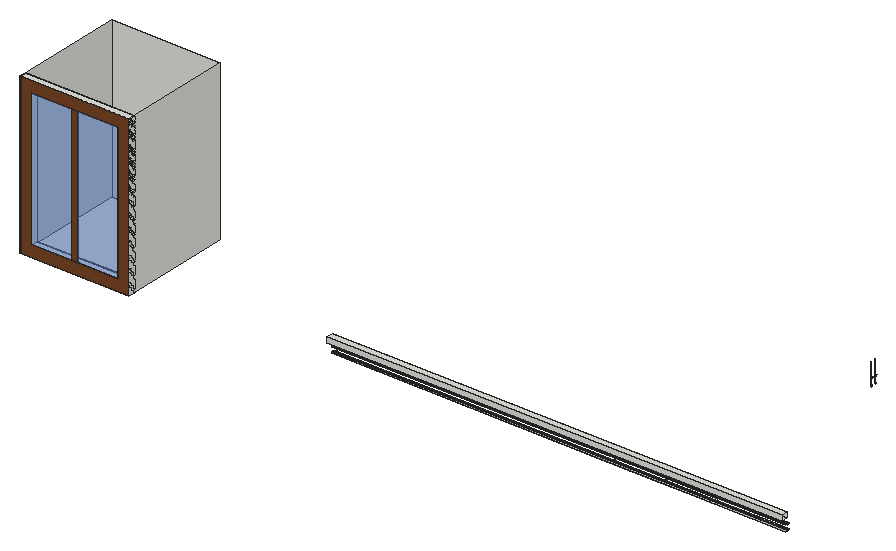
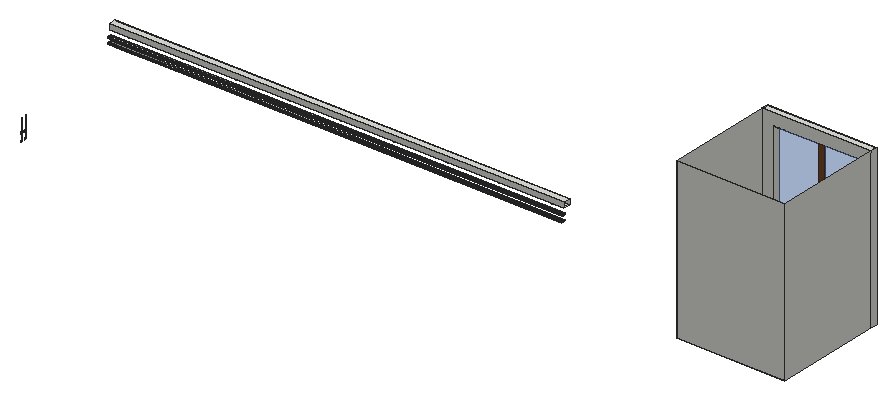
# SketchUp Ruby script. Lengths in inches.
U = 1.inch
M = Sketchup.active_model
def pt(a) = Geom::Point3d.new(a.map { |v| v * U })
def face(e, loops, mat)
  f = e.add_face(loops[0].map { |a| pt(a) })
  loops[1..].each { |l| e.add_face(l.map { |a| pt(a) }).erase! }
  f.material = f.back_material = mat if mat
  f
end
# faces: each face lists its corners as indices into pts; further lists are holes
def faces(e, pts, list, mat = nil) = list.each { |f| face(e, (f[0].is_a?(Array) ? f : [f]).map { |l| l.map { |i| pts[i] } }, mat) }
# xy, xz, yz: faces in a plane at the given z, y or x. An outline is a flat list of corners, or four numbers for a rectangle; further outlines are holes
def ring(l) = l.size == 4 ? [[l[0], l[1]], [l[2], l[1]], [l[2], l[3]], [l[0], l[3]]] : l.each_slice(2).to_a
def flat(e, list, mat, &to3) = list.each { |f| face(e, (f[0].is_a?(Array) ? f : [f]).map { |l| ring(l).map { |u, v| to3.(u, v) } }, mat) }
def xy(e, z, list, mat = nil) = flat(e, list, mat) { |x, y| [x, y, z] }
def xz(e, y, list, mat = nil) = flat(e, list, mat) { |x, z| [x, y, z] }
def yz(e, x, list, mat = nil) = flat(e, list, mat) { |y, z| [x, y, z] }
def lines(e, pts, list) = list.each { |a, b| e.add_line(pt(pts[a]), pt(pts[b])) }
# prism: a flat outline (further loops are holes) pulled along v
def prism(e, loops, v, mat = nil)
  f = face(e, loops, mat); d = Geom::Vector3d.new(v.map { |x| x * U })
  f.pushpull(f.normal.samedirection?(d) ? d.length : -d.length)
end
def box(e, o, s, mat = nil) = prism(e, [[o, [o[0] + s[0], o[1], o[2]], [o[0] + s[0], o[1] + s[1], o[2]], [o[0], o[1] + s[1], o[2]]]], [0, 0, s[2]], mat)
def at(x, y, z, deg = 0) = Geom::Transformation.translation(pt([x, y, z])) * Geom::Transformation.rotation(ORIGIN, Z_AXIS, deg.degrees)
def axes(o, x, y, z) = Geom::Transformation.new([*x, 0, *y, 0, *z, 0, *pt(o).to_a, 1])
def part(name) = M.definitions.add(name)
# library, detail: a bought-in or finely detailed component or shape, given as its bounding box
def library(name, o, s) = part(name).tap { |d| box(d.entities, o, s) }
def detail(e, o, s) = box(e.add_group.entities, o, s)
def put(e, d, t, mat = nil) = e.add_instance(d, t).tap { |i| i.material = mat if mat }
def group(e, t, mat = nil) = e.add_group.tap { |g| g.transformation = t; g.material = mat if mat }.entities
root = M.entities
M.materials.add("Material \#1").color = [140, 140, 140]
M.materials.add("[Translucent Glass Blue]").color = [100, 149, 237]
M.materials["[Translucent Glass Blue]"].alpha = 0.5
M.materials.add("[Wood Veneer 01]").color = [120, 70, 37]
xy(root,150.179,[[115.793,121.25,154.87,162.1875]])
xy(root,150.749,[[220.539,130.192,320.53,130.817],[320.53,130.192,338.843,130.817],[338.843,130.192,359.155,130.817]])
xy(root,151.187,[[220.539,130.192,320.53,130.817],[320.53,130.192,338.843,130.817]])
xy(root,152.749,[[220.539,130.192,320.53,130.817],[320.53,130.192,338.843,130.817],[338.843,130.192,359.155,130.817]])
xy(root,153.187,[[220.539,130.192,320.53,130.817],[320.53,130.192,338.843,130.817]])
xy(root,155.037,[[[220.539,128.022,383.845,130.647],[357.535,128.645,357.794,128.679,358.035,128.779,358.242,128.9375,358.401,129.145,358.501,129.386,358.535,129.645,358.501,129.904,358.401,130.145,358.242,130.352,358.035,130.511,357.794,130.611,357.535,130.645,357.276,130.611,357.035,130.511,356.828,130.352,356.669,130.145,356.569,129.904,356.535,129.645,356.569,129.386,356.669,129.145,356.828,128.9375,357.035,128.779,357.276,128.679],[338.535,128.645,338.794,128.679,339.035,128.779,339.242,128.9375,339.401,129.145,339.501,129.386,339.535,129.645,339.501,129.904,339.401,130.145,339.242,130.352,339.035,130.511,338.794,130.611,338.535,130.645,338.276,130.611,338.035,130.511,337.828,130.352,337.669,130.145,337.569,129.904,337.535,129.645,337.569,129.386,337.669,129.145,337.828,128.9375,338.035,128.779,338.276,128.679],[319.535,128.645,319.794,128.679,320.035,128.779,320.242,128.9375,320.401,129.145,320.501,129.386,320.535,129.645,320.501,129.904,320.401,130.145,320.242,130.352,320.035,130.511,319.794,130.611,319.535,130.645,319.276,130.611,319.035,130.511,318.828,130.352,318.669,130.145,318.569,129.904,318.535,129.645,318.569,129.386,318.669,129.145,318.828,128.9375,319.035,128.779,319.276,128.679],[300.535,128.645,300.794,128.679,301.035,128.779,301.242,128.9375,301.401,129.145,301.501,129.386,301.535,129.645,301.501,129.904,301.401,130.145,301.242,130.352,301.035,130.511,300.794,130.611,300.535,130.645,300.276,130.611,300.035,130.511,299.828,130.352,299.669,130.145,299.569,129.904,299.535,129.645,299.569,129.386,299.669,129.145,299.828,128.9375,300.035,128.779,300.276,128.679],[281.535,128.645,281.794,128.679,282.035,128.779,282.242,128.9375,282.401,129.145,282.501,129.386,282.535,129.645,282.501,129.904,282.401,130.145,282.242,130.352,282.035,130.511,281.794,130.611,281.535,130.645,281.276,130.611,281.035,130.511,280.828,130.352,280.669,130.145,280.569,129.904,280.535,129.645,280.569,129.386,280.669,129.145,280.828,128.9375,281.035,128.779,281.276,128.679],[262.535,128.645,262.794,128.679,263.035,128.779,263.242,128.9375,263.401,129.145,263.501,129.386,263.535,129.645,263.501,129.904,263.401,130.145,263.242,130.352,263.035,130.511,262.794,130.611,262.535,130.645,262.276,130.611,262.035,130.511,261.828,130.352,261.669,130.145,261.569,129.904,261.535,129.645,261.569,129.386,261.669,129.145,261.828,128.9375,262.035,128.779,262.276,128.679],[243.535,128.645,243.794,128.679,244.035,128.779,244.242,128.9375,244.401,129.145,244.501,129.386,244.535,129.645,244.501,129.904,244.401,130.145,244.242,130.352,244.035,130.511,243.794,130.611,243.535,130.645,243.276,130.611,243.035,130.511,242.828,130.352,242.669,130.145,242.569,129.904,242.535,129.645,242.569,129.386,242.669,129.145,242.828,128.9375,243.035,128.779,243.276,128.679],[224.535,128.645,224.794,128.679,225.035,128.779,225.242,128.9375,225.401,129.145,225.501,129.386,225.535,129.645,225.501,129.904,225.401,130.145,225.242,130.352,225.035,130.511,224.794,130.611,224.535,130.645,224.276,130.611,224.035,130.511,223.828,130.352,223.669,130.145,223.569,129.904,223.535,129.645,223.569,129.386,223.669,129.145,223.828,128.9375,224.035,128.779,224.276,128.679],[376.66,128.645,376.919,128.679,377.16,128.779,377.367,128.9375,377.526,129.145,377.626,129.386,377.66,129.645,377.626,129.904,377.526,130.145,377.367,130.352,377.16,130.511,376.919,130.611,376.66,130.645,376.401,130.611,376.16,130.511,375.953,130.352,375.794,130.145,375.694,129.904,375.66,129.645,375.694,129.386,375.794,129.145,375.953,128.9375,376.16,128.779,376.401,128.679]]])
xy(root,156.974,[[220.539,128.022,383.845,130.647]])
xz(root,128.022,[[220.539,155.037,383.845,156.974]])
xz(root,130.192,[[220.539,150.749,383.845,151.187],[220.539,152.749,383.845,153.187]])
xz(root,130.647,[[220.539,155.037,383.845,156.974]])
xz(root,130.817,[[220.539,151.062,320.53,151.187],[320.53,151.062,338.843,151.187],[338.843,151.062,359.155,151.187],[220.539,153.062,320.53,153.187],[320.53,153.062,338.843,153.187],
  [338.843,153.062,359.155,153.187]])
xz(root,131.35,[[220.539,150.725,383.845,151.037],[220.539,152.725,383.845,153.037]])
xz(root,162.1875,[[115.793,150.179,154.87,207.139]])
xz(root,199.277,[[359.415,161.063,359.412,161.068,359.318,161.238],[359.412,161.068,359.408,161.073,359.318,161.238],[359.408,161.073,359.363,161.122,359.318,161.238],[359.408,161.073,359.404,161.077,359.363,161.122],[359.404,161.077,359.382,161.098,359.363,161.122],
  [359.363,161.122,359.334,161.176,359.318,161.238],[359.363,161.122,359.347,161.148,359.334,161.176],[359.39,161.133,359.318,161.238,359.365,161.174],[359.365,161.174,359.318,161.238,359.349,161.221],[359.334,161.176,359.324,161.206,359.318,161.238],
  [359.349,161.221,359.318,161.238,359.344,161.271],[359.318,161.238,359.316,161.271,359.323,161.328],[359.318,161.238,359.323,161.328,359.368,161.427],[359.318,161.238,359.349,161.322,359.344,161.271],[359.318,161.238,359.368,161.427,359.349,161.322],
  [359.349,161.322,359.368,161.427,359.365,161.368],[359.323,161.328,359.34,161.381,359.368,161.427],[359.365,161.368,359.368,161.427,359.39,161.409],[359.39,161.409,359.368,161.427,359.422,161.443],[359.368,161.427,359.404,161.466,359.448,161.495],
  [359.368,161.427,359.46,161.469,359.422,161.443]],"Material \#1")
xz(root,199.308,[[359.443,158.434,359.341,158.464,359.444,158.445],[359.444,158.445,359.341,158.464,359.344,158.475],[359.341,158.464,359.247,158.512,359.344,158.475],[359.344,158.475,359.247,158.512,359.252,158.521],[359.247,158.512,359.162,158.575,359.252,158.521],
  [359.252,158.521,359.162,158.575,359.169,158.584],[359.162,158.575,359.089,158.653,359.169,158.584],[359.169,158.584,359.089,158.653,359.097,158.66],[359.089,158.653,359.033,158.737,359.097,158.66],[359.429,158.655,359.398,158.672,359.406,158.679],
  [359.097,158.66,359.033,158.737,359.042,158.743],[359.398,158.672,359.378,158.702,359.406,158.679],[359.406,158.679,359.378,158.702,359.387,158.707],[359.378,158.702,359.363,158.735,359.387,158.707],[359.387,158.707,359.363,158.735,359.373,158.739],
  [359.363,158.735,359.354,158.771,359.373,158.739],[359.033,158.737,358.985,158.842,359.042,158.743],[359.373,158.739,359.354,158.771,359.364,158.773],[359.042,158.743,358.985,158.842,358.995,158.846],[359.354,158.771,359.351,158.806,359.364,158.773],
  [359.364,158.773,359.351,158.806,359.361,158.806],[359.351,158.806,359.354,158.848,359.361,158.806],[359.361,158.806,359.354,158.848,359.364,158.846],[358.985,158.842,358.957,158.951,358.995,158.846],[358.995,158.846,358.957,158.951,358.967,158.953],
  [359.364,158.846,359.354,158.848,359.363,158.884],[359.364,158.846,359.363,158.884,359.373,158.88],[359.373,158.88,359.363,158.884,359.378,158.917],[359.373,158.88,359.378,158.917,359.387,158.912],[359.387,158.912,359.378,158.917,359.398,158.947],
  [359.387,158.912,359.398,158.947,359.406,158.94],[359.406,158.94,359.398,158.947,359.422,158.973],[358.957,158.951,358.947,159.071,358.967,158.953],[358.967,158.953,358.947,159.071,358.957,159.071],[358.947,159.071,358.947,166.411,358.957,159.071],
  [358.957,159.071,358.947,166.411,358.957,166.41]],"Material \#1")
xz(root,199.588,[[359.415,161.063,359.318,161.238,359.412,161.068],[359.415,161.063,359.365,161.174,359.318,161.238],[359.415,161.063,359.39,161.133,359.365,161.174],[359.412,161.068,359.318,161.238,359.408,161.073],[359.408,161.073,359.318,161.238,359.363,161.122],
  [359.408,161.073,359.363,161.122,359.404,161.077],[359.404,161.077,359.363,161.122,359.382,161.098],[359.363,161.122,359.318,161.238,359.334,161.176],[359.363,161.122,359.334,161.176,359.347,161.148],[359.365,161.174,359.349,161.221,359.318,161.238],
  [359.334,161.176,359.318,161.238,359.324,161.206],[359.349,161.221,359.344,161.271,359.318,161.238],[359.318,161.238,359.323,161.328,359.316,161.271],[359.318,161.238,359.344,161.271,359.349,161.322],[359.318,161.238,359.349,161.322,359.365,161.368],
  [359.318,161.238,359.365,161.368,359.368,161.427],[359.318,161.238,359.368,161.427,359.323,161.328],[359.323,161.328,359.368,161.427,359.34,161.381],[359.365,161.368,359.39,161.409,359.368,161.427],[359.39,161.409,359.422,161.443,359.368,161.427],
  [359.368,161.427,359.448,161.495,359.404,161.466]],"Material \#1")
xz(root,200.833,[[359.415,161.063,359.318,161.238,359.365,161.174],[359.415,161.063,359.412,161.068,359.318,161.238],[359.415,161.063,359.365,161.174,359.39,161.133],[359.412,161.068,359.408,161.073,359.318,161.238],[359.408,161.073,359.363,161.122,359.318,161.238],
  [359.408,161.073,359.404,161.077,359.363,161.122],[359.404,161.077,359.382,161.098,359.363,161.122],[359.363,161.122,359.334,161.176,359.318,161.238],[359.363,161.122,359.347,161.148,359.334,161.176],[359.365,161.174,359.318,161.238,359.349,161.221],
  [359.334,161.176,359.324,161.206,359.318,161.238],[359.349,161.221,359.318,161.238,359.344,161.271],[359.318,161.238,359.316,161.271,359.323,161.328],[359.318,161.238,359.323,161.328,359.368,161.427],[359.318,161.238,359.349,161.322,359.344,161.271],
  [359.318,161.238,359.365,161.368,359.349,161.322],[359.318,161.238,359.368,161.427,359.365,161.368],[359.323,161.328,359.34,161.381,359.368,161.427],[359.365,161.368,359.368,161.427,359.39,161.409],[359.39,161.409,359.368,161.427,359.422,161.443],
  [359.368,161.427,359.404,161.466,359.448,161.495]],"Material \#1")
xz(root,201.113,[[359.443,158.434,359.444,158.445,359.341,158.464],[359.444,158.445,359.344,158.475,359.341,158.464],[359.341,158.464,359.344,158.475,359.247,158.512],[359.344,158.475,359.252,158.521,359.247,158.512],[359.247,158.512,359.252,158.521,359.162,158.575],
  [359.252,158.521,359.169,158.584,359.162,158.575],[359.162,158.575,359.169,158.584,359.089,158.653],[359.169,158.584,359.097,158.66,359.089,158.653],[359.089,158.653,359.097,158.66,359.033,158.737],[359.429,158.655,359.406,158.679,359.398,158.672],
  [359.097,158.66,359.042,158.743,359.033,158.737],[359.398,158.672,359.406,158.679,359.378,158.702],[359.406,158.679,359.387,158.707,359.378,158.702],[359.378,158.702,359.387,158.707,359.363,158.735],[359.387,158.707,359.373,158.739,359.363,158.735],
  [359.363,158.735,359.373,158.739,359.354,158.771],[359.033,158.737,359.042,158.743,358.985,158.842],[359.373,158.739,359.364,158.773,359.354,158.771],[359.042,158.743,358.995,158.846,358.985,158.842],[359.354,158.771,359.364,158.773,359.351,158.806],
  [359.364,158.773,359.361,158.806,359.351,158.806],[359.351,158.806,359.361,158.806,359.354,158.848],[359.361,158.806,359.364,158.846,359.354,158.848],[358.985,158.842,358.995,158.846,358.957,158.951],[358.995,158.846,358.967,158.953,358.957,158.951],
  [359.364,158.846,359.363,158.884,359.354,158.848],[359.364,158.846,359.373,158.88,359.363,158.884],[359.373,158.88,359.378,158.917,359.363,158.884],[359.373,158.88,359.387,158.912,359.378,158.917],[359.387,158.912,359.398,158.947,359.378,158.917],
  [359.387,158.912,359.406,158.94,359.398,158.947],[359.406,158.94,359.422,158.973,359.398,158.947],[358.957,158.951,358.967,158.953,358.947,159.071],[358.967,158.953,358.957,159.071,358.947,159.071],[358.947,159.071,358.957,159.071,358.947,166.411],
  [358.957,159.071,358.957,166.41,358.947,166.411]],"Material \#1")
xz(root,201.144,[[359.415,161.063,359.318,161.238,359.412,161.068],[359.412,161.068,359.318,161.238,359.408,161.073],[359.408,161.073,359.318,161.238,359.363,161.122],[359.408,161.073,359.363,161.122,359.404,161.077],[359.404,161.077,359.363,161.122,359.382,161.098],
  [359.363,161.122,359.318,161.238,359.334,161.176],[359.363,161.122,359.334,161.176,359.347,161.148],[359.39,161.133,359.365,161.174,359.318,161.238],[359.365,161.174,359.349,161.221,359.318,161.238],[359.334,161.176,359.318,161.238,359.324,161.206],
  [359.349,161.221,359.344,161.271,359.318,161.238],[359.318,161.238,359.323,161.328,359.316,161.271],[359.318,161.238,359.344,161.271,359.349,161.322],[359.318,161.238,359.349,161.322,359.368,161.427],[359.318,161.238,359.368,161.427,359.323,161.328],
  [359.349,161.322,359.365,161.368,359.368,161.427],[359.323,161.328,359.368,161.427,359.34,161.381],[359.365,161.368,359.39,161.409,359.368,161.427],[359.39,161.409,359.422,161.443,359.368,161.427],[359.368,161.427,359.448,161.495,359.404,161.466]],"Material \#1")
yz(root,115.793,[[121.25,150.179,162.1875,207.139]])
yz(root,154.87,[[121.25,150.179,162.1875,207.139]])
p = [[378.845,130.817,150.749],[359.155,130.817,150.749],[338.843,130.817,150.749],[320.53,130.817,150.749],[220.539,130.817,150.749],[220.539,131.35,150.725],
  [320.53,131.35,150.725],[338.843,131.35,150.725],[359.155,131.35,150.725],[378.845,131.35,150.725],[383.845,131.35,150.725],[383.845,130.817,150.749],
  [320.53,131.35,151.037],[220.539,131.35,151.037],[220.539,131.355,151.162],[320.53,131.355,151.162],[338.843,131.35,151.037],[338.843,131.355,151.162],
  [359.155,131.35,151.037],[359.155,131.355,151.162],[220.539,130.817,151.062],[320.53,130.817,151.062],[320.53,130.823,151.187],[220.539,130.823,151.187],
  [338.843,130.817,151.062],[338.843,130.823,151.187],[359.155,130.817,151.062],[359.155,130.823,151.187],[378.845,130.823,151.187],[383.845,130.823,151.187],
  [383.845,131.355,151.162],[378.845,131.355,151.162],[383.845,131.35,152.725],[383.845,130.817,152.749],[378.845,130.817,152.749],[359.155,130.817,152.749],
  [338.843,130.817,152.749],[320.53,130.817,152.749],[220.539,130.817,152.749],[220.539,131.35,152.725],[320.53,131.35,152.725],[338.843,131.35,152.725],
  [359.155,131.35,152.725],[378.845,131.35,152.725],[320.53,131.35,153.037],[220.539,131.35,153.037],[220.539,131.355,153.162],[320.53,131.355,153.162],
  [338.843,131.35,153.037],[338.843,131.355,153.162],[359.155,131.35,153.037],[359.155,131.355,153.162],[220.539,130.817,153.062],[320.53,130.817,153.062],
  [320.53,130.823,153.187],[220.539,130.823,153.187],[338.843,130.817,153.062],[338.843,130.823,153.187],[359.155,130.817,153.062],[359.155,130.823,153.187],
  [378.845,131.355,153.162],[378.845,130.823,153.187],[383.845,130.823,153.187],[383.845,131.355,153.162],[357.535,129.645,155.465],[338.41,129.645,155.465],
  [319.285,129.645,155.465],[300.16,129.645,155.465],[281.035,129.645,155.465],[261.91,129.645,155.465],[242.785,129.645,155.465],[223.66,129.645,155.465],
  [220.539,129.645,155.465],[359.155,130.965,152.898],[338.843,130.965,152.898],[320.53,130.965,152.898],[220.539,130.965,152.898],[359.155,130.965,150.898],
  [338.843,130.965,150.898],[320.53,130.965,150.898],[220.539,130.965,150.898]]
faces(root,p,[[0,1,2,3,4,5,6,7,8,9,10,11],[12,13,14,15],[16,12,15,17],[18,16,17,19],[20,21,22,23],[21,24,25,22],[24,26,27,25],[17,15,14,23,22,25,27,28,29,30,31,19],
  [32,33,34,35,36,37,38,39,40,41,42,43],[44,45,46,47],[48,44,47,49],[50,48,49,51],[52,53,54,55],[53,56,57,54],[56,58,59,57],[60,51,49,47,46,55,54,57,59,61,62,63]])
lines(root,p,[[64,65],[65,66],[66,67],[67,68],[68,69],[69,70],[70,71],[71,72],[73,74],[74,75],[75,76],[77,78],
  [79,80],[78,79]])
g1 = group(root,at(115.79,121.25,150.18))
xy(g1,0,[[0,0,39.08,2.375]])
xy(g1,4.11,[[4.11,0,34.97,2.375]])
xy(g1,52.85,[[4.11,0,34.97,2.375]])
xy(g1,56.96,[[0,0,39.08,2.375]])
xz(g1,0,[[4.11,4.11,18.54,52.85],[20.54,4.11,34.97,52.85]],"[Translucent Glass Blue]")
xz(g1,0,[[[0,0,39.08,56.96],[4.11,4.11,34.97,52.85]],[18.54,4.11,20.54,52.85]],"[Wood Veneer 01]")
xz(g1,2.375,[[[0,0,39.08,56.96],[4.11,4.11,34.97,52.85]]])
yz(g1,0,[[0,0,2.375,56.96]])
yz(g1,4.11,[[0,4.11,2.375,52.85]])
yz(g1,34.97,[[0,4.11,2.375,52.85]])
yz(g1,39.08,[[0,0,2.375,56.96]])
